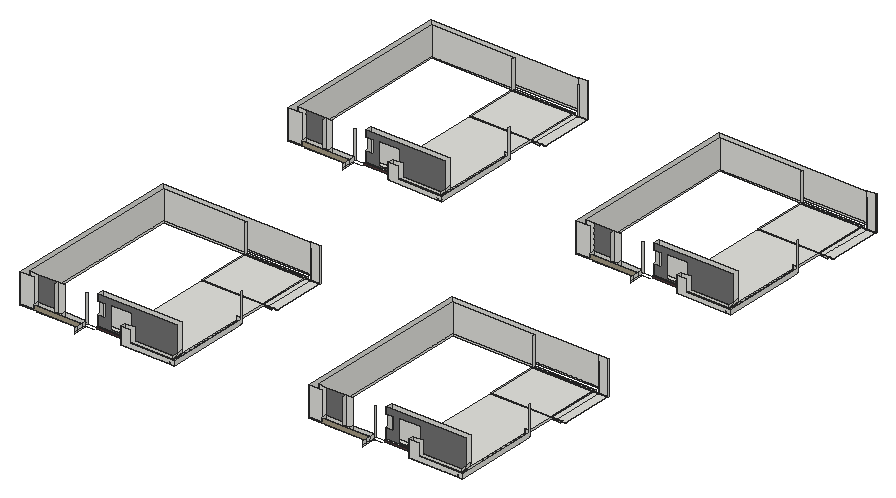
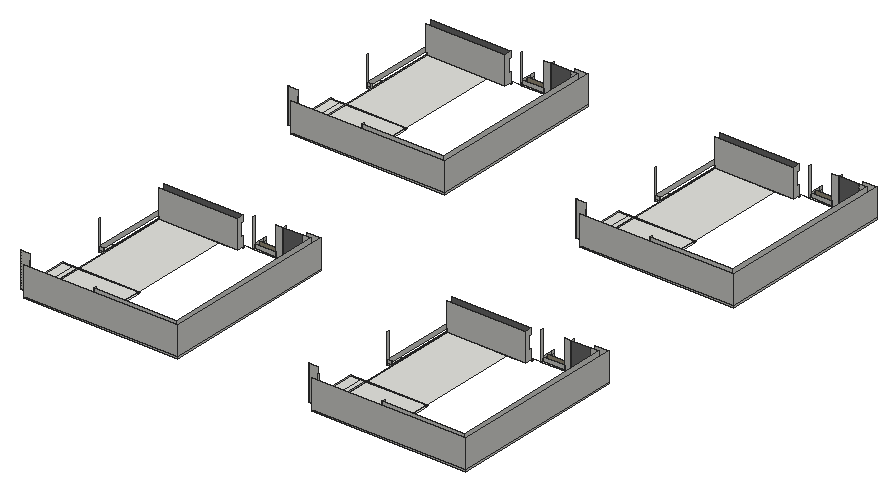
# SketchUp Ruby script. Lengths in inches.
U = 1.inch
M = Sketchup.active_model
def pt(a) = Geom::Point3d.new(a.map { |v| v * U })
def face(e, loops, mat)
  f = e.add_face(loops[0].map { |a| pt(a) })
  loops[1..].each { |l| e.add_face(l.map { |a| pt(a) }).erase! }
  f.material = f.back_material = mat if mat
  f
end
# faces: each face lists its corners as indices into pts; further lists are holes
def faces(e, pts, list, mat = nil) = list.each { |f| face(e, (f[0].is_a?(Array) ? f : [f]).map { |l| l.map { |i| pts[i] } }, mat) }
# xy, xz, yz: faces in a plane at the given z, y or x. An outline is a flat list of corners, or four numbers for a rectangle; further outlines are holes
def ring(l) = l.size == 4 ? [[l[0], l[1]], [l[2], l[1]], [l[2], l[3]], [l[0], l[3]]] : l.each_slice(2).to_a
def flat(e, list, mat, &to3) = list.each { |f| face(e, (f[0].is_a?(Array) ? f : [f]).map { |l| ring(l).map { |u, v| to3.(u, v) } }, mat) }
def xy(e, z, list, mat = nil) = flat(e, list, mat) { |x, y| [x, y, z] }
def xz(e, y, list, mat = nil) = flat(e, list, mat) { |x, z| [x, y, z] }
def yz(e, x, list, mat = nil) = flat(e, list, mat) { |y, z| [x, y, z] }
def lines(e, pts, list) = list.each { |a, b| e.add_line(pt(pts[a]), pt(pts[b])) }
# prism: a flat outline (further loops are holes) pulled along v
def prism(e, loops, v, mat = nil)
  f = face(e, loops, mat); d = Geom::Vector3d.new(v.map { |x| x * U })
  f.pushpull(f.normal.samedirection?(d) ? d.length : -d.length)
end
def box(e, o, s, mat = nil) = prism(e, [[o, [o[0] + s[0], o[1], o[2]], [o[0] + s[0], o[1] + s[1], o[2]], [o[0], o[1] + s[1], o[2]]]], [0, 0, s[2]], mat)
def at(x, y, z, deg = 0) = Geom::Transformation.translation(pt([x, y, z])) * Geom::Transformation.rotation(ORIGIN, Z_AXIS, deg.degrees)
def axes(o, x, y, z) = Geom::Transformation.new([*x, 0, *y, 0, *z, 0, *pt(o).to_a, 1])
def part(name) = M.definitions.add(name)
# library, detail: a bought-in or finely detailed component or shape, given as its bounding box
def library(name, o, s) = part(name).tap { |d| box(d.entities, o, s) }
def detail(e, o, s) = box(e.add_group.entities, o, s)
def put(e, d, t, mat = nil) = e.add_instance(d, t).tap { |i| i.material = mat if mat }
def group(e, t, mat = nil) = e.add_group.tap { |g| g.transformation = t; g.material = mat if mat }.entities
root = M.entities
M.materials.add("[Color M05]").color = [114, 114, 114]
M.materials.add("[Concrete Tile]").color = [165, 155, 133]
M.materials.add("[Granite Brown]").color = [89, 59, 61]
xy(root,756,[[333.89,1799.9375,333.89,1822.9375,402.4,1822.9375,402.4,1806.5625,431.33,1806.5625,431.33,1822.9375,523.04,1822.9375,523.04,1799.9375],[686.87,1799.9375,686.87,1822.9375,852.25,1822.9375,852.25,1812.1875,857.6875,1812.1875,857.6875,1822.9375,890.875,1822.9375,890.875,1833.5,894.3125,1833.5,894.3125,1799.9375],[894.3125,1799.9375,913.875,1800.6875],[1552.08,1799.9375,1552.08,1822.9375,1620.59,1822.9375,1620.59,1806.5625,1649.52,1806.5625,1649.52,1822.9375,1741.23,1822.9375,1741.23,1799.9375],[1905.06,1799.9375,1905.06,1822.9375,2070.4375,1822.9375,2070.4375,1812.1875,2075.875,1812.1875,2075.875,1822.9375,2109.0625,1822.9375,2109.0625,1833.5,2112.5,1833.5,2112.5,1799.9375],
  [2112.5,1799.9375,2132.0625,1800.6875],[852.25,1812.1875,857.6875,1822.9375],[2070.4375,1812.1875,2075.875,1822.9375],[686.87,1822.9375,686.87,1833.5,648.68,1833.5,648.68,1837.0625,847.6875,1837.0625,847.6875,1834.4375,852.25,1834.4375,852.25,1822.9375],[852.25,1822.9375,857.6875,2091.0625],
  [857.6875,1822.9375,890.875,1833.5],[1905.06,1822.9375,1905.06,1833.5,1866.87,1833.5,1866.87,1837.0625,2065.875,1837.0625,2065.875,1834.4375,2070.4375,1834.4375,2070.4375,1822.9375],[2070.4375,1822.9375,2075.875,2091.0625],[2075.875,1822.9375,2109.0625,1833.5],[557.88,1833.5,557.88,1835.1875,557.4,1835.1875,557.4,1837.0625,648.68,1837.0625,648.68,1833.5],
  [857.6875,1833.5,890.875,1834.4375],[890.875,1833.5,894.3125,2091.0625],[1776.07,1833.5,1776.07,1835.1875,1775.59,1835.1875,1775.59,1837.0625,1866.87,1837.0625,1866.87,1833.5],[2075.875,1833.5,2109.0625,1834.4375],[2109.0625,1833.5,2112.5,2091.0625],
  [847.6875,1834.4375,852.25,2091.0625],[857.6875,1834.4375,890.875,2091.0625],[2065.875,1834.4375,2070.4375,2091.0625],[2075.875,1834.4375,2109.0625,2091.0625],[894.3125,2091.0625,913.875,2148.83],
  [2112.5,2091.0625,2132.0625,2148.83],[635.3125,2290,890.875,2295.875],[1853.5,2290,2109.0625,2295.875],[635.3125,2295.875,890.875,2518.89],[890.875,2295.875,913.875,2518.89],
  [1853.5,2295.875,2109.0625,2518.89],[2109.0625,2295.875,2132.0625,2518.89],[333.89,3214.625,333.89,3237.625,402.4,3237.625,402.4,3221.25,431.33,3221.25,431.33,3237.625,523.04,3237.625,523.04,3214.625],[686.87,3214.625,686.87,3237.625,852.25,3237.625,852.25,3226.875,857.6875,3226.875,857.6875,3237.625,890.875,3237.625,890.875,3248.1875,894.3125,3248.1875,894.3125,3214.625],[894.3125,3214.625,913.875,3215.375],
  [1552.08,3214.625,1552.08,3237.625,1620.59,3237.625,1620.59,3221.25,1649.52,3221.25,1649.52,3237.625,1741.23,3237.625,1741.23,3214.625],[1905.06,3214.625,1905.06,3237.625,2070.4375,3237.625,2070.4375,3226.875,2075.875,3226.875,2075.875,3237.625,2109.0625,3237.625,2109.0625,3248.1875,2112.5,3248.1875,2112.5,3214.625],[2112.5,3214.625,2132.0625,3215.375],[852.25,3226.875,857.6875,3237.625],[2070.4375,3226.875,2075.875,3237.625],
  [686.87,3237.625,686.87,3248.1875,648.68,3248.1875,648.68,3251.75,847.6875,3251.75,847.6875,3249.125,852.25,3249.125,852.25,3237.625],[852.25,3237.625,857.6875,3505.75],[857.6875,3237.625,890.875,3248.1875],[1905.06,3237.625,1905.06,3248.1875,1866.87,3248.1875,1866.87,3251.75,2065.875,3251.75,2065.875,3249.125,2070.4375,3249.125,2070.4375,3237.625],[2070.4375,3237.625,2075.875,3505.75],
  [2075.875,3237.625,2109.0625,3248.1875],[557.88,3248.1875,557.88,3249.875,557.4,3249.875,557.4,3251.75,648.68,3251.75,648.68,3248.1875],[857.6875,3248.1875,890.875,3249.125],[890.875,3248.1875,894.3125,3505.75],[1776.07,3248.1875,1776.07,3249.875,1775.59,3249.875,1775.59,3251.75,1866.87,3251.75,1866.87,3248.1875],
  [2075.875,3248.1875,2109.0625,3249.125],[2109.0625,3248.1875,2112.5,3505.75],[847.6875,3249.125,852.25,3505.75],[857.6875,3249.125,890.875,3505.75],[2065.875,3249.125,2070.4375,3505.75],
  [2075.875,3249.125,2109.0625,3505.75],[894.3125,3505.75,913.875,3563.51],[2112.5,3505.75,2132.0625,3563.51],[635.3125,3704.6875,890.875,3710.5625],[1853.5,3704.6875,2109.0625,3710.5625],
  [635.3125,3710.5625,890.875,3933.57],[890.875,3710.5625,913.875,3933.57],[1853.5,3710.5625,2109.0625,3933.57],[2109.0625,3710.5625,2132.0625,3933.57]])
xy(root,762,[[686.87,1822.9375,890.875,1822.9375,890.875,1842.5,635.3125,1842.5,635.3125,1833.5,686.87,1833.5],[1905.06,1822.9375,2109.0625,1822.9375,2109.0625,1842.5,1853.5,1842.5,1853.5,1833.5,1905.06,1833.5],[557.88,1833.5,635.3125,1842.5],[1776.07,1833.5,1853.5,1842.5],[557.4,1842.5,635.3125,1869.5],
  [635.3125,1842.5,890.875,1869.5],[894,1842.5,894.3125,2148.83],[1775.59,1842.5,1853.5,1869.5],[1853.5,1842.5,2109.0625,1869.5],[2112.1875,1842.5,2112.5,2148.83],
  [635.3125,1869.5,890.875,2295.875],[1853.5,1869.5,2109.0625,2295.875],[894,2148.83,894.3125,2156.01],[894.3125,2148.83,913.875,2156.01],[2112.1875,2148.83,2112.5,2156.01],
  [2112.5,2148.83,2132.0625,2156.01],[635.3125,2295.875,890.875,2518.89],[890.875,2295.875,913.875,2518.89],[913.875,2295.875,954.6875,2518.89],[1853.5,2295.875,2109.0625,2518.89],
  [2109.0625,2295.875,2132.0625,2518.89],[2132.0625,2295.875,2172.875,2518.89],[635.3125,2518.89,890.875,2531.375],[913.875,2518.89,954.6875,2520.14],[1853.5,2518.89,2109.0625,2531.375],
  [2132.0625,2518.89,2172.875,2520.14],[686.87,3237.625,890.875,3237.625,890.875,3257.1875,635.3125,3257.1875,635.3125,3248.1875,686.87,3248.1875],[1905.06,3237.625,2109.0625,3237.625,2109.0625,3257.1875,1853.5,3257.1875,1853.5,3248.1875,1905.06,3248.1875],[557.88,3248.1875,635.3125,3257.1875],[1776.07,3248.1875,1853.5,3257.1875],
  [557.4,3257.1875,635.3125,3284.1875],[635.3125,3257.1875,890.875,3284.1875],[894,3257.1875,894.3125,3563.51],[1775.59,3257.1875,1853.5,3284.1875],[1853.5,3257.1875,2109.0625,3284.1875],
  [2112.1875,3257.1875,2112.5,3563.51],[635.3125,3284.1875,890.875,3710.5625],[1853.5,3284.1875,2109.0625,3710.5625],[894,3563.51,894.3125,3570.7],[894.3125,3563.51,913.875,3570.7],
  [2112.1875,3563.51,2112.5,3570.7],[2112.5,3563.51,2132.0625,3570.7],[635.3125,3710.5625,890.875,3933.57],[890.875,3710.5625,913.875,3933.57],[913.875,3710.5625,954.6875,3933.57],
  [1853.5,3710.5625,2109.0625,3933.57],[2109.0625,3710.5625,2132.0625,3933.57],[2132.0625,3710.5625,2172.875,3933.57],[635.3125,3933.57,890.875,3946.0625],[913.875,3933.57,954.6875,3934.82],
  [1853.5,3933.57,2109.0625,3946.0625],[2132.0625,3933.57,2172.875,3934.82]])
xy(root,762.0625,[[686.18,1799.9375,686.87,1822.9375],[1904.37,1799.9375,1905.06,1822.9375],[686.18,3214.625,686.87,3237.625],[1904.37,3214.625,1905.06,3237.625]])
xz(root,1799.9375,[[262.875,756,319.53,762],[686.87,756,913.875,756,913.875,774.75,727.43,774.75,727.43,825,686.18,825,686.18,762.0625,686.87,762.0625],[1481.0625,756,1537.72,762],[1905.06,756,2132.0625,756,2132.0625,774.75,1945.62,774.75,1945.62,825,1904.37,825,1904.37,762.0625,1905.06,762.0625],[262.875,762,319.53,882],
  [1481.0625,762,1537.72,882]])
xz(root,1799.9375,[[319.53,756,523.04,777.4375],[1537.72,756,1741.23,777.4375]],"[Concrete Tile]")
xz(root,1806.5625,[[402.43,762,402.43,777.4375,402.51,777.4375],[402.43,762,431.33,762,431.33,777.4375,402.51,777.4375],[1620.62,762,1620.62,777.4375,1620.7,777.4375],[1620.62,762,1649.52,762,1649.52,777.4375,1620.7,777.4375]])
xz(root,1822.9375,[[387.59,756,387.59,756.07,402.4,756],[686.87,756,890.875,762],[1605.78,756,1605.78,756.07,1620.59,756],[1905.06,756,2109.0625,762],[285.875,762,319.53,882],
  [319.53,762,402.43,777.4375],[402.43,762,403.03,882,431.33,882,431.33,762],[431.33,762,523.04,777.4375],[686.87,762,890.875,762.0625],[1504.0625,762,1537.72,882],
  [1537.72,762,1620.62,777.4375],[1620.62,762,1621.22,882,1649.52,882,1649.52,762],[1649.52,762,1741.23,777.4375],[1905.06,762,2109.0625,762.0625],[686.18,762.0625,686.18,825,727.43,825,727.43,774.75,890.875,774.75,890.875,762.0625],
  [1904.37,762.0625,1904.37,825,1945.62,825,1945.62,774.75,2109.0625,774.75,2109.0625,762.0625]])
xz(root,1822.9375,[[402.43,762,403.03,882,319.53,882,319.53,777.4375,402.43,777.4375],[1620.62,762,1621.22,882,1537.72,882,1537.72,777.4375,1620.62,777.4375]],"[Color M05]")
xz(root,1833.5,[[557.88,756,686.87,762],[1776.07,756,1905.06,762]],"[Granite Brown]")
xz(root,1842.5,[[890.875,762,894.3125,762.0625],[2109.0625,762,2112.5,762.0625]])
xz(root,1842.5,[[[557.88,762,890.875,762,890.875,774.75,891.6875,774.75,891.6875,882,557.88,882,557.88,857.4,589.71,857.4,589.71,805.12,557.88,805.12],[632.49,763.875,632.49,764.1875,611.65,764.1875,611.65,862,701.59,862,701.59,763.875]],[[1776.07,762,2109.0625,762,2109.0625,774.75,2109.875,774.75,2109.875,882,1776.07,882,1776.07,857.4,1807.9,857.4,1807.9,805.12,1776.07,805.12],[1850.67,763.875,1850.67,764.1875,1829.84,764.1875,1829.84,862,1919.77,862,1919.77,763.875]]],"[Color M05]")
xz(root,1842.5,[[557.4,762,557.88,805.12],[1775.59,762,1776.07,805.12]],"[Granite Brown]")
xz(root,1869.5,[[557.4,762,557.4,882,891.6875,882,891.6875,774.75,890.875,774.75,890.875,762],[1775.59,762,1775.59,882,2109.875,882,2109.875,774.75,2109.0625,774.75,2109.0625,762]])
xz(root,2148.83,[[894.3125,756,913.875,762],[2112.5,756,2132.0625,762]])
xz(root,2156.01,[[894.3125,756,913.875,762],[2112.5,756,2132.0625,762],[894,762,894.3125,779.36],[894.3125,762,913.875,779.36],[2112.1875,762,2112.5,779.36],
  [2112.5,762,2132.0625,779.36]])
xz(root,2295.875,[[913.875,756,930.75,762],[2132.0625,756,2148.9375,762],[635.3125,762,890.875,763.75],[890.875,762,913.875,763.75],[913.875,762,930.75,763.75],
  [930.75,762,954.6875,763.75],[1853.5,762,2109.0625,763.75],[2109.0625,762,2132.0625,763.75],[2132.0625,762,2148.9375,763.75],[2148.9375,762,2172.875,763.75]])
xz(root,2518.89,[[635.3125,762,890.875,763.75],[890.875,762,913.875,763.75],[913.875,762,954.6875,763.75],[1853.5,762,2109.0625,763.75],[2109.0625,762,2132.0625,763.75],
  [2132.0625,762,2172.875,763.75]])
xz(root,2520.14,[[913.875,762,954.6875,908.8125],[2132.0625,762,2172.875,908.8125]])
xz(root,2531.375,[[285.875,756,890.875,762],[1504.0625,756,2109.0625,762],[285.875,762,635.3125,882],[1504.0625,762,1853.5,882]])
xz(root,2554.375,[[262.875,756,913.875,762],[1481.0625,756,2132.0625,762],[262.875,762,913.875,882],[1481.0625,762,2132.0625,882]])
xz(root,3214.625,[[262.875,756,319.53,762],[686.87,756,913.875,756,913.875,774.75,727.43,774.75,727.43,825,686.18,825,686.18,762.0625,686.87,762.0625],[1481.0625,756,1537.72,762],[1905.06,756,2132.0625,756,2132.0625,774.75,1945.62,774.75,1945.62,825,1904.37,825,1904.37,762.0625,1905.06,762.0625],[262.875,762,319.53,882],
  [1481.0625,762,1537.72,882]])
xz(root,3214.625,[[319.53,756,523.04,777.4375],[1537.72,756,1741.23,777.4375]],"[Concrete Tile]")
xz(root,3221.25,[[402.43,762,402.43,777.4375,402.51,777.4375],[402.43,762,431.33,762,431.33,777.4375,402.51,777.4375],[1620.62,762,1620.62,777.4375,1620.7,777.4375],[1620.62,762,1649.52,762,1649.52,777.4375,1620.7,777.4375]])
xz(root,3237.625,[[387.59,756,387.59,756.07,402.4,756],[686.87,756,890.875,762],[1605.78,756,1605.78,756.07,1620.59,756],[1905.06,756,2109.0625,762],[285.875,762,319.53,882],
  [319.53,762,402.43,777.4375],[402.43,762,403.03,882,431.33,882,431.33,762],[431.33,762,523.04,777.4375],[686.87,762,890.875,762.0625],[1504.0625,762,1537.72,882],
  [1537.72,762,1620.62,777.4375],[1620.62,762,1621.22,882,1649.52,882,1649.52,762],[1649.52,762,1741.23,777.4375],[1905.06,762,2109.0625,762.0625],[686.18,762.0625,686.18,825,727.43,825,727.43,774.75,890.875,774.75,890.875,762.0625],
  [1904.37,762.0625,1904.37,825,1945.62,825,1945.62,774.75,2109.0625,774.75,2109.0625,762.0625]])
xz(root,3237.625,[[402.43,762,403.03,882,319.53,882,319.53,777.4375,402.43,777.4375],[1620.62,762,1621.22,882,1537.72,882,1537.72,777.4375,1620.62,777.4375]],"[Color M05]")
xz(root,3248.1875,[[557.88,756,686.87,762],[1776.07,756,1905.06,762]],"[Granite Brown]")
xz(root,3257.1875,[[890.875,762,894.3125,762.0625],[2109.0625,762,2112.5,762.0625]])
xz(root,3257.1875,[[[557.88,762,890.875,762,890.875,774.75,891.6875,774.75,891.6875,882,557.88,882,557.88,857.4,589.71,857.4,589.71,805.12,557.88,805.12],[632.49,763.875,632.49,764.1875,611.65,764.1875,611.65,862,701.59,862,701.59,763.875]],[[1776.07,762,2109.0625,762,2109.0625,774.75,2109.875,774.75,2109.875,882,1776.07,882,1776.07,857.4,1807.9,857.4,1807.9,805.12,1776.07,805.12],[1850.67,763.875,1850.67,764.1875,1829.84,764.1875,1829.84,862,1919.77,862,1919.77,763.875]]],"[Color M05]")
xz(root,3257.1875,[[557.4,762,557.88,805.12],[1775.59,762,1776.07,805.12]],"[Granite Brown]")
xz(root,3284.1875,[[557.4,762,557.4,882,891.6875,882,891.6875,774.75,890.875,774.75,890.875,762],[1775.59,762,1775.59,882,2109.875,882,2109.875,774.75,2109.0625,774.75,2109.0625,762]])
xz(root,3563.51,[[894.3125,756,913.875,762],[2112.5,756,2132.0625,762]])
xz(root,3570.7,[[894.3125,756,913.875,762],[2112.5,756,2132.0625,762],[894,762,894.3125,779.36],[894.3125,762,913.875,779.36],[2112.1875,762,2112.5,779.36],
  [2112.5,762,2132.0625,779.36]])
xz(root,3710.5625,[[913.875,756,930.75,762],[2132.0625,756,2148.9375,762],[635.3125,762,890.875,763.75],[890.875,762,913.875,763.75],[913.875,762,930.75,763.75],
  [930.75,762,954.6875,763.75],[1853.5,762,2109.0625,763.75],[2109.0625,762,2132.0625,763.75],[2132.0625,762,2148.9375,763.75],[2148.9375,762,2172.875,763.75]])
xz(root,3933.57,[[635.3125,762,890.875,763.75],[890.875,762,913.875,763.75],[913.875,762,954.6875,763.75],[1853.5,762,2109.0625,763.75],[2109.0625,762,2132.0625,763.75],
  [2132.0625,762,2172.875,763.75]])
xz(root,3934.82,[[913.875,762,954.6875,908.8125],[2132.0625,762,2172.875,908.8125]])
xz(root,3946.0625,[[285.875,756,890.875,762],[1504.0625,756,2109.0625,762],[285.875,762,635.3125,882],[1504.0625,762,1853.5,882]])
xz(root,3969.0625,[[262.875,756,913.875,762],[1481.0625,756,2132.0625,762],[262.875,762,913.875,882],[1481.0625,762,2132.0625,882]])
yz(root,262.875,[[1799.9375,756,2554.375,762],[3214.625,756,3969.0625,762],[1799.9375,762,2554.375,882],[3214.625,762,3969.0625,882]])
yz(root,285.875,[[1822.9375,756,2531.375,762],[3237.625,756,3946.0625,762],[1822.9375,762,2531.375,882],[3237.625,762,3946.0625,882]])
yz(root,319.53,[[1799.9375,762,1822.9375,777.4375],[3214.625,762,3237.625,777.4375]])
yz(root,402.43,[[1806.5625,762,1822.9375,777.4375],[3221.25,762,3237.625,777.4375]])
yz(root,431.33,[[1806.5625,762,1822.9375,777.4375],[3221.25,762,3237.625,777.4375]])
yz(root,523.04,[[1763.25,756,1799.9375,762],[3177.9375,756,3214.625,762],[1763.25,762,1799.9375,777.4375],[1799.9375,762,1822.9375,777.4375],[1822.9375,762,1830.25,882],
  [3177.9375,762,3214.625,777.4375],[3214.625,762,3237.625,777.4375],[3237.625,762,3244.9375,882]])
yz(root,557.4,[[1842.5,762,1842.5,805.12,1853.125,805.12,1853.125,857.4,1842.5,857.4,1842.5,882,1869.5,882,1869.5,762],[3257.1875,762,3257.1875,805.12,3267.8125,805.12,3267.8125,857.4,3257.1875,857.4,3257.1875,882,3284.1875,882,3284.1875,762]])
yz(root,635.3125,[[2295.875,762,2518.89,763.75],[2518.89,762,2531.375,882],[3710.5625,762,3933.57,763.75],[3933.57,762,3946.0625,882]])
yz(root,686.18,[[1799.9375,762.0625,1822.9375,825],[3214.625,762.0625,3237.625,825]])
yz(root,686.87,[[1799.9375,756,1822.9375,762.0625],[1822.9375,756,1833.5,762],[3214.625,756,3237.625,762.0625],[3237.625,756,3248.1875,762]])
yz(root,890.875,[[1822.9375,756,2531.375,762],[3237.625,756,3946.0625,762],[1822.9375,762,1842.5,762.0625],[1842.5,762,1869.5,762.0625],[2295.875,762,2518.89,763.75],
  [3237.625,762,3257.1875,762.0625],[3257.1875,762,3284.1875,762.0625],[3710.5625,762,3933.57,763.75],[1822.9375,762.0625,1842.5,774.75],[1842.5,762.0625,1869.5,774.75],
  [3237.625,762.0625,3257.1875,774.75],[3257.1875,762.0625,3284.1875,774.75]])
yz(root,894.3125,[[1800.6875,756,1842.5,762],[2148.83,756,2156.01,762],[3215.375,756,3257.1875,762],[3563.51,756,3570.7,762]])
yz(root,913.875,[[1799.9375,756,2148.83,756,2148.83,762,2156.01,762,2156.01,882,2148.83,882,2148.83,774.75,1799.9375,774.75],[2148.83,756,2156.01,762],[3214.625,756,3563.51,756,3563.51,762,3570.7,762,3570.7,882,3563.51,882,3563.51,774.75,3214.625,774.75],[3563.51,756,3570.7,762],[2518.89,762,2520.14,882],
  [3933.57,762,3934.82,882]])
yz(root,954.6875,[[2295.875,762,2518.89,763.75],[2518.89,762,2520.14,908.8125],[3710.5625,762,3933.57,763.75],[3933.57,762,3934.82,908.8125]])
yz(root,1481.0625,[[1799.9375,756,2554.375,762],[3214.625,756,3969.0625,762],[1799.9375,762,2554.375,882],[3214.625,762,3969.0625,882]])
yz(root,1504.0625,[[1822.9375,756,2531.375,762],[3237.625,756,3946.0625,762],[1822.9375,762,2531.375,882],[3237.625,762,3946.0625,882]])
yz(root,1537.72,[[1799.9375,762,1822.9375,777.4375],[3214.625,762,3237.625,777.4375]])
yz(root,1620.62,[[1806.5625,762,1822.9375,777.4375],[3221.25,762,3237.625,777.4375]])
yz(root,1649.52,[[1806.5625,762,1822.9375,777.4375],[3221.25,762,3237.625,777.4375]])
yz(root,1741.23,[[1763.25,756,1799.9375,762],[3177.9375,756,3214.625,762],[1763.25,762,1799.9375,777.4375],[1799.9375,762,1822.9375,777.4375],[1822.9375,762,1830.25,882],
  [3177.9375,762,3214.625,777.4375],[3214.625,762,3237.625,777.4375],[3237.625,762,3244.9375,882]])
yz(root,1775.59,[[1842.5,762,1842.5,805.12,1853.125,805.12,1853.125,857.4,1842.5,857.4,1842.5,882,1869.5,882,1869.5,762],[3257.1875,762,3257.1875,805.12,3267.8125,805.12,3267.8125,857.4,3257.1875,857.4,3257.1875,882,3284.1875,882,3284.1875,762]])
yz(root,1853.5,[[2295.875,762,2518.89,763.75],[2518.89,762,2531.375,882],[3710.5625,762,3933.57,763.75],[3933.57,762,3946.0625,882]])
yz(root,1904.37,[[1799.9375,762.0625,1822.9375,825],[3214.625,762.0625,3237.625,825]])
yz(root,1905.06,[[1799.9375,756,1822.9375,762.0625],[1822.9375,756,1833.5,762],[3214.625,756,3237.625,762.0625],[3237.625,756,3248.1875,762]])
yz(root,2109.0625,[[1822.9375,756,2531.375,762],[3237.625,756,3946.0625,762],[1822.9375,762,1842.5,762.0625],[1842.5,762,1869.5,762.0625],[2295.875,762,2518.89,763.75],
  [3237.625,762,3257.1875,762.0625],[3257.1875,762,3284.1875,762.0625],[3710.5625,762,3933.57,763.75],[1822.9375,762.0625,1842.5,774.75],[1842.5,762.0625,1869.5,774.75],
  [3237.625,762.0625,3257.1875,774.75],[3257.1875,762.0625,3284.1875,774.75]])
yz(root,2112.5,[[1800.6875,756,1842.5,762],[2148.83,756,2156.01,762],[3215.375,756,3257.1875,762],[3563.51,756,3570.7,762]])
yz(root,2132.0625,[[1799.9375,756,2148.83,756,2148.83,762,2156.01,762,2156.01,882,2148.83,882,2148.83,774.75,1799.9375,774.75],[2148.83,756,2156.01,762],[3214.625,756,3563.51,756,3563.51,762,3570.7,762,3570.7,882,3563.51,882,3563.51,774.75,3214.625,774.75],[3563.51,756,3570.7,762],[2518.89,762,2520.14,882],
  [3933.57,762,3934.82,882]])
yz(root,2172.875,[[2295.875,762,2518.89,763.75],[2518.89,762,2520.14,908.8125],[3710.5625,762,3933.57,763.75],[3933.57,762,3934.82,908.8125]])
p = [[402.4,1806.5625,756],[402.4,1822.9375,756],[387.59,1822.9375,756.07],[387.59,1806.5625,756.07],[1620.59,1806.5625,756],[1620.59,1822.9375,756],
  [1605.78,1822.9375,756.07],[1605.78,1806.5625,756.07],[402.4,3221.25,756],[402.4,3237.625,756],[387.59,3237.625,756.07],[387.59,3221.25,756.07],
  [1620.59,3221.25,756],[1620.59,3237.625,756],[1605.78,3237.625,756.07],[1605.78,3221.25,756.07],[402.43,1822.9375,762],[402.43,1806.5625,762],
  [402.51,1806.5625,777.4375],[403.03,1806.5625,882],[403.03,1822.9375,882],[1620.62,1822.9375,762],[1620.62,1806.5625,762],[1620.7,1806.5625,777.4375],
  [1621.22,1806.5625,882],[1621.22,1822.9375,882],[402.43,3237.625,762],[402.43,3221.25,762],[402.51,3221.25,777.4375],[403.03,3221.25,882],
  [403.03,3237.625,882],[1620.62,3237.625,762],[1620.62,3221.25,762],[1620.7,3221.25,777.4375],[1621.22,3221.25,882],[1621.22,3237.625,882],
  [1741.23,1822.9375,756],[1775.59,1822.9375,756],[1741.23,1830.25,762],[1775.59,1830.25,762],[1853.5,1830.25,762],[1853.5,1833.5,762],
  [2109.0625,1822.9375,762.0625],[2109.0625,1799.9375,762.0625],[2112.1875,1842.5,762],[2112.1875,1799.9375,762],[2132.0625,1800.6875,762],[2112.5,1800.6875,762],
  [1741.23,1778.3125,762],[1741.23,1778.3125,777.4375],[1741.23,1778.3125,756],[523.04,1822.9375,756],[557.4,1822.9375,756],[523.04,1830.25,762],
  [557.4,1830.25,762],[635.3125,1830.25,762],[635.3125,1833.5,762],[890.875,1822.9375,762.0625],[890.875,1799.9375,762.0625],[894,1842.5,762],
  [894,1799.9375,762],[913.875,1800.6875,762],[894.3125,1800.6875,762],[523.04,1778.3125,756],[523.04,1778.3125,762],[523.04,1778.3125,777.4375],
  [1741.23,3237.625,756],[1775.59,3237.625,756],[1741.23,3193,756],[1741.23,3193,762],[1741.23,3193,777.4375],[2109.0625,3237.625,762.0625],
  [2109.0625,3214.625,762.0625],[2132.0625,3215.375,762],[2112.5,3215.375,762],[2112.1875,3257.1875,762],[2112.1875,3214.625,762],[1741.23,3244.9375,762],
  [1775.59,3244.9375,762],[1853.5,3244.9375,762],[1853.5,3248.1875,762],[890.875,3237.625,762.0625],[890.875,3214.625,762.0625],[894,3257.1875,762],
  [894,3214.625,762],[913.875,3215.375,762],[894.3125,3215.375,762],[523.04,3244.9375,762],[557.4,3244.9375,762],[635.3125,3244.9375,762],
  [635.3125,3248.1875,762],[523.04,3237.625,756],[557.4,3237.625,756],[523.04,3193,756],[523.04,3193,762],[523.04,3193,777.4375]]
faces(root,p,[[0,1,2,3],[4,5,6,7],[8,9,10,11],[12,13,14,15],[16,17,18,19,20],[21,22,23,24,25],[26,27,28,29,30],[31,32,33,34,35]])
lines(root,p,[[36,37],[38,39],[40,41],[42,43],[44,45],[46,47],[48,49],[50,48],[51,52],[53,54],[55,56],[57,58],
  [59,60],[61,62],[63,64],[64,65],[66,67],[68,69],[69,70],[71,72],[73,74],[75,76],[77,78],[79,80],
  [81,82],[83,84],[85,86],[87,88],[89,90],[91,92],[93,94],[94,95]])
